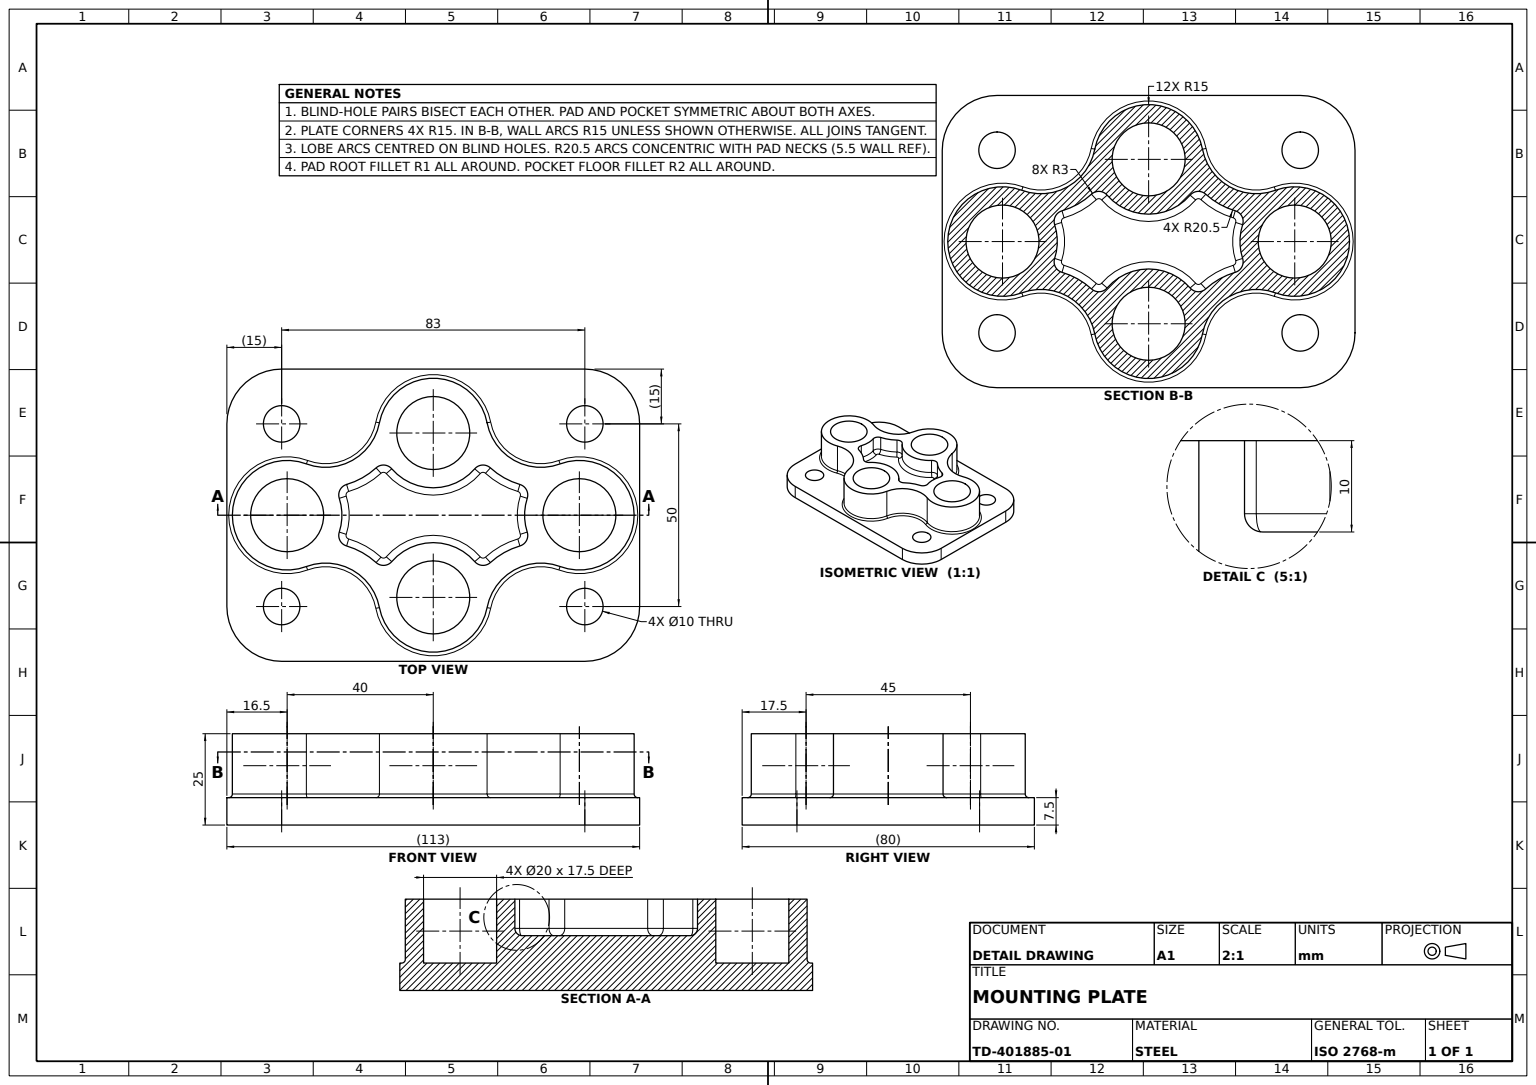
solid
v1 (14.982821,-34.38617,7.5)
v2 (-14.982821,-34.38617,7.5)
e1 v1 v2 CIRCLE(AX(P(0,-40,7.5),D(0,0,1),D(1,0,0)),16) rev
v3 (14.046394,-34.737034,8.5)
e2 v1 v3 CIRCLE(AX(P(14.982821,-34.38617,8.5),D(-0.350864382,0.936426284,0),D(-0.936426284,-0.350864382,0)),1)
v4 (-14.046394,-34.737034,8.5)
e3 v4 v3 CIRCLE(AX(P(0,-40,8.5),D(0,0,1),D(1,0,0)),15)
e4 v2 v4 CIRCLE(AX(P(-14.982821,-34.38617,8.5),D(-0.350864382,-0.936426284,0),D(0.936426284,-0.350864382,0)),1)
face TORUS(AX(P(0,-40,8.5),D(0,0,1),D(1,0,0)),16,1) rev [-e1 e2 -e3 -e4]
v5 (-40,41.5,7.5)
v6 (-40,-41.5,7.5)
e5 v5 v6 LINE
v7 (-40,41.5,0)
e6 v5 v7 LINE
v8 (-40,-41.5,0)
e7 v7 v8 LINE
e8 v8 v6 LINE
face PLANE(AX(P(-40,56.5,7.5),D(1,0,0),D(0,1,0))) rev [-e5 e6 e7 e8]
v9 (40,41.5,7.5)
v10 (25,56.5,7.5)
e9 v9 v10 CIRCLE(AX(P(25,41.5,7.5),D(0,0,1),D(1,0,0)),15)
v11 (40,41.5,0)
e10 v11 v9 LINE
v12 (25,56.5,0)
e11 v12 v11 CIRCLE(AX(P(25,41.5,0),D(0,0,1),D(1,0,0)),15) rev
e12 v10 v12 LINE
face CYL(AX(P(25,41.5,7.5),D(0,0,-1),D(-1,0,0)),15) [-e9 -e10 -e11 -e12]
v13 (-25.296394,-14.737034,8.5)
e13 v13 v4 CIRCLE(AX(P(-28.092789,-29.474069,8.5),D(0,0,1),D(1,0,0)),15) rev
v14 (-14.046394,-34.737034,25)
e14 v14 v4 LINE
v15 (-25.296394,-14.737034,25)
e15 v15 v14 CIRCLE(AX(P(-28.092789,-29.474069,25),D(0,0,-1),D(1,0,0)),15)
e16 v15 v13 LINE
face CYL(AX(P(-28.092789,-29.474069,25),D(0,0,-1),D(-1,0,0)),15) rev [e13 -e14 -e15 e16]
v16 (14.046394,-34.737034,25)
e17 v16 v3 LINE
e18 v14 v16 CIRCLE(AX(P(0,-40,25),D(0,0,1),D(1,0,0)),15)
face CYL(AX(P(0,-40,25),D(0,0,-1),D(-1,0,0)),15) [-e17 -e18 e14 e3]
v17 (-5.231122,23.824853,15)
v18 (-4.615696,25.727812,17)
e19 v17 v18 CIRCLE(AX(P(-5.231122,23.824853,17),D(0.95147921,-0.307713037,0),D(0.307713037,0.95147921,0)),2)
v19 (5.231122,23.824853,15)
e20 v19 v17 CIRCLE(AX(P(0,40,15),D(0,0,1),D(1,0,0)),17) rev
v20 (4.615696,25.727812,17)
e21 v19 v20 CIRCLE(AX(P(5.231122,23.824853,17),D(0.95147921,0.307713037,0),D(-0.307713037,0.95147921,0)),2)
e22 v18 v20 CIRCLE(AX(P(0,40,17),D(0,0,1),D(1,0,0)),15)
face TORUS(AX(P(0,40,17),D(0,0,1),D(1,0,0)),17,2) rev [-e19 -e20 e21 -e22]
v21 (-12.699871,11.355944,17)
v22 (-12.955115,15.650146,17)
e23 v21 v22 CIRCLE(AX(P(-10.739845,13.627133,17),D(0,0,1),D(1,0,0)),3) rev
v23 (-11.393187,12.87007,15)
e24 v23 v21 CIRCLE(AX(P(-11.393187,12.87007,17),D(-0.757062957,0.653341932,0),D(-0.653341932,-0.757062957,0)),2)
v24 (-11.478268,14.301471,15)
e25 v24 v23 CIRCLE(AX(P(-10.739845,13.627133,15),D(0,0,1),D(1,0,0)),1)
e26 v24 v22 CIRCLE(AX(P(-11.478268,14.301471,17),D(0.674337673,0.738423119,0),D(-0.738423119,0.674337673,0)),2)
face DEGENERATE_TOROIDAL_SURFACE(AX(P(-10.739845,13.627133,17),D(0,0,1),D(1,0,0)),1,2,.T.) rev [-e23 -e24 -e25 e26]
v25 (12.955115,-15.650146,17)
v26 (12.955115,-15.650146,25)
e27 v25 v26 LINE
v27 (12.699871,-11.355944,25)
e28 v27 v26 CIRCLE(AX(P(10.739845,-13.627133,25),D(0,0,1),D(1,0,0)),3) rev
v28 (12.699871,-11.355944,17)
e29 v28 v27 LINE
e30 v28 v25 CIRCLE(AX(P(10.739845,-13.627133,17),D(0,0,1),D(1,0,0)),3) rev
face CYL(AX(P(10.739845,-13.627133,43),D(0,0,-1),D(-1,0,0)),3) rev [e27 -e28 -e29 e30]
v29 (20,-41.5,7.5)
e31 v29 v29 CIRCLE(AX(P(25,-41.5,7.5),D(0,0,-1),D(-1,0,0)),5)
v30 (30,-41.5,0)
e32 v30 v30 CIRCLE(AX(P(25,-41.5,0),D(0,0,1),D(1,0,0)),5)
face CYL(AX(P(25,-41.5,7.5),D(0,0,-1),D(-1,0,0)),5) rev [-e31] [-e32]
v31 (25,-56.5,7.5)
v32 (40,-41.5,7.5)
e33 v31 v32 CIRCLE(AX(P(25,-41.5,7.5),D(0,0,1),D(1,0,0)),15)
v33 (25,-56.5,0)
e34 v33 v31 LINE
v34 (40,-41.5,0)
e35 v34 v33 CIRCLE(AX(P(25,-41.5,0),D(0,0,1),D(1,0,0)),15) rev
e36 v32 v34 LINE
face CYL(AX(P(25,-41.5,7.5),D(0,0,-1),D(-1,0,0)),15) [-e33 -e34 -e35 -e36]
v35 (-8.418063,-23.716016,17)
v36 (-12.955115,-15.650146,17)
e37 v35 v36 CIRCLE(AX(P(-28.092789,-29.474069,17),D(0,0,1),D(1,0,0)),20.5)
v37 (-6.498577,-23.154255,15)
e38 v35 v37 CIRCLE(AX(P(-6.498577,-23.154255,17),D(0.280880609,-0.959742717,0),D(0.959742717,0.280880609,0)),2)
v38 (-11.478268,-14.301471,15)
e39 v38 v37 CIRCLE(AX(P(-28.092789,-29.474069,15),D(0,0,1),D(1,0,0)),22.5) rev
e40 v36 v38 CIRCLE(AX(P(-11.478268,-14.301471,17),D(0.674337673,-0.738423119,0),D(0.738423119,0.674337673,0)),2)
face TORUS(AX(P(-28.092789,-29.474069,17),D(0,0,1),D(1,0,0)),22.5,2) rev [-e37 e38 -e39 -e40]
v39 (8.418063,-23.716016,17)
v40 (4.615696,-25.727812,17)
e41 v39 v40 CIRCLE(AX(P(5.538835,-22.873374,17),D(0,0,1),D(1,0,0)),3) rev
v41 (4.615696,-25.727812,25)
e42 v40 v41 LINE
v42 (8.418063,-23.716016,25)
e43 v42 v41 CIRCLE(AX(P(5.538835,-22.873374,25),D(0,0,1),D(1,0,0)),3) rev
e44 v39 v42 LINE
face CYL(AX(P(5.538835,-22.873374,43),D(0,0,-1),D(-1,0,0)),3) rev [e41 e42 -e43 -e44]
v43 (25.482821,-15.719503,7.5)
e45 v43 v1 CIRCLE(AX(P(28.092789,-29.474069,7.5),D(0,0,1),D(1,0,0)),14)
v44 (25.296394,-14.737034,8.5)
e46 v43 v44 CIRCLE(AX(P(25.482821,-15.719503,8.5),D(0.982468951,0.186426284,0),D(-0.186426284,0.982468951,0)),1)
e47 v3 v44 CIRCLE(AX(P(28.092789,-29.474069,8.5),D(0,0,1),D(1,0,0)),15) rev
face TORUS(AX(P(28.092789,-29.474069,8.5),D(0,0,1),D(1,0,0)),14,1) rev [-e2 -e45 e46 -e47]
v45 (-25.482821,15.719503,7.5)
v46 (-14.982821,34.38617,7.5)
e48 v45 v46 CIRCLE(AX(P(-28.092789,29.474069,7.5),D(0,0,1),D(1,0,0)),14)
v47 (-25.296394,14.737034,8.5)
e49 v47 v45 CIRCLE(AX(P(-25.482821,15.719503,8.5),D(0.982468951,0.186426284,0),D(-0.186426284,0.982468951,0)),1)
v48 (-14.046394,34.737034,8.5)
e50 v48 v47 CIRCLE(AX(P(-28.092789,29.474069,8.5),D(0,0,1),D(1,0,0)),15) rev
e51 v48 v46 CIRCLE(AX(P(-14.982821,34.38617,8.5),D(-0.350864382,0.936426284,0),D(-0.936426284,-0.350864382,0)),1)
face TORUS(AX(P(-28.092789,29.474069,8.5),D(0,0,1),D(1,0,0)),14,1) rev [-e48 -e49 -e50 e51]
v49 (30,41.5,0)
e52 v49 v49 CIRCLE(AX(P(25,41.5,0),D(0,0,1),D(1,0,0)),5)
v50 (20,41.5,7.5)
e53 v50 v50 CIRCLE(AX(P(25,41.5,7.5),D(0,0,-1),D(-1,0,0)),5)
face CYL(AX(P(25,41.5,7.5),D(0,0,-1),D(-1,0,0)),5) rev [-e52] [-e53]
v51 (-11.393187,-12.87007,15)
e54 v51 v38 CIRCLE(AX(P(-10.739845,-13.627133,15),D(0,0,1),D(1,0,0)),1)
v52 (-12.699871,-11.355944,17)
e55 v51 v52 CIRCLE(AX(P(-11.393187,-12.87007,17),D(0.757062957,0.653341932,0),D(-0.653341932,0.757062957,0)),2)
e56 v36 v52 CIRCLE(AX(P(-10.739845,-13.627133,17),D(0,0,1),D(1,0,0)),3) rev
face DEGENERATE_TOROIDAL_SURFACE(AX(P(-10.739845,-13.627133,17),D(0,0,1),D(1,0,0)),1,2,.T.) rev [e40 -e54 e55 -e56]
v53 (14.982821,34.38617,7.5)
v54 (25.482821,15.719503,7.5)
e57 v53 v54 CIRCLE(AX(P(28.092789,29.474069,7.5),D(0,0,1),D(1,0,0)),14)
v55 (14.046394,34.737034,8.5)
e58 v55 v53 CIRCLE(AX(P(14.982821,34.38617,8.5),D(-0.350864382,-0.936426284,0),D(0.936426284,-0.350864382,0)),1)
v56 (25.296394,14.737034,8.5)
e59 v56 v55 CIRCLE(AX(P(28.092789,29.474069,8.5),D(0,0,1),D(1,0,0)),15) rev
e60 v54 v56 CIRCLE(AX(P(25.482821,15.719503,8.5),D(-0.982468951,0.186426284,0),D(-0.186426284,-0.982468951,0)),1)
face TORUS(AX(P(28.092789,29.474069,8.5),D(0,0,1),D(1,0,0)),14,1) rev [-e57 -e58 -e59 -e60]
v57 (-8.418063,23.716016,17)
e61 v57 v18 CIRCLE(AX(P(-5.538835,22.873374,17),D(0,0,1),D(1,0,0)),3) rev
v58 (-6.498577,23.154255,15)
e62 v58 v57 CIRCLE(AX(P(-6.498577,23.154255,17),D(0.280880609,0.959742717,0),D(-0.959742717,0.280880609,0)),2)
e63 v17 v58 CIRCLE(AX(P(-5.538835,22.873374,15),D(0,0,1),D(1,0,0)),1)
face DEGENERATE_TOROIDAL_SURFACE(AX(P(-5.538835,22.873374,17),D(0,0,1),D(1,0,0)),1,2,.T.) rev [e19 -e61 -e62 -e63]
v59 (-25.296394,14.737034,25)
e64 v59 v15 CIRCLE(AX(P(-22.5,0,25),D(0,0,1),D(1,0,0)),15)
e65 v59 v47 LINE
e66 v47 v13 CIRCLE(AX(P(-22.5,0,8.5),D(0,0,1),D(1,0,0)),15)
face CYL(AX(P(-22.5,0,25),D(0,0,-1),D(-1,0,0)),15) [-e64 e65 e66 -e16]
v60 (-25,56.5,0)
e67 v7 v60 CIRCLE(AX(P(-25,41.5,0),D(0,0,1),D(1,0,0)),15) rev
v61 (-25,56.5,7.5)
e68 v61 v5 CIRCLE(AX(P(-25,41.5,7.5),D(0,0,1),D(1,0,0)),15)
e69 v60 v61 LINE
face CYL(AX(P(-25,41.5,7.5),D(0,0,-1),D(-1,0,0)),15) [-e67 -e6 -e68 -e69]
v62 (12.699871,11.355944,17)
e70 v62 v28 CIRCLE(AX(P(22.5,0,17),D(0,0,1),D(1,0,0)),15)
v63 (12.699871,11.355944,25)
e71 v63 v27 CIRCLE(AX(P(22.5,0,25),D(0,0,1),D(1,0,0)),15)
e72 v62 v63 LINE
face CYL(AX(P(22.5,0,43),D(0,0,-1),D(-1,0,0)),15) [e70 e29 -e71 -e72]
v64 (-25,-56.5,7.5)
v65 (-25,-56.5,0)
e73 v64 v65 LINE
e74 v65 v33 LINE
e75 v64 v31 LINE
face PLANE(AX(P(-40,-56.5,7.5),D(0,1,0),D(0,0,1))) rev [e73 e74 e34 -e75]
e76 v10 v61 LINE
e77 v12 v60 LINE
face PLANE(AX(P(40,56.5,7.5),D(0,-1,0),D(0,0,-1))) rev [-e76 e12 e77 e69]
v66 (-20,-41.5,0)
e78 v66 v66 CIRCLE(AX(P(-25,-41.5,0),D(0,0,1),D(1,0,0)),5)
v67 (-20,41.5,0)
e79 v67 v67 CIRCLE(AX(P(-25,41.5,0),D(0,0,1),D(1,0,0)),5)
e80 v34 v11 LINE
e81 v65 v8 CIRCLE(AX(P(-25,-41.5,0),D(0,0,1),D(1,0,0)),15) rev
face PLANE(AX(P(-25.296394,-14.737034,0),D(0,0,1),D(1,0,0))) rev [e78] [e52] [e32] [e79] [e11 -e80 e35 -e74 e81 -e7 e67 -e77]
v68 (-10,-40,7.5)
e82 v68 v68 CIRCLE(AX(P(0,-40,7.5),D(0,0,-1),D(-1,0,0)),10) rev
face PLANE(AX(P(0,-40,7.5),D(0,0,-1),D(-1,0,0))) rev [e82]
v69 (-4.615696,25.727812,25)
v70 (4.615696,25.727812,25)
e83 v69 v70 CIRCLE(AX(P(0,40,25),D(0,0,1),D(1,0,0)),15)
e84 v18 v69 LINE
e85 v20 v70 LINE
face CYL(AX(P(0,40,43),D(0,0,-1),D(-1,0,0)),15) [-e83 -e84 e22 e85]
v71 (12.955115,15.650146,17)
e86 v71 v62 CIRCLE(AX(P(10.739845,13.627133,17),D(0,0,1),D(1,0,0)),3) rev
v72 (12.955115,15.650146,25)
e87 v72 v63 CIRCLE(AX(P(10.739845,13.627133,25),D(0,0,1),D(1,0,0)),3) rev
e88 v71 v72 LINE
face CYL(AX(P(10.739845,13.627133,43),D(0,0,-1),D(-1,0,0)),3) rev [e86 e72 -e87 -e88]
v73 (25.296394,14.737034,25)
v74 (14.046394,34.737034,25)
e89 v73 v74 CIRCLE(AX(P(28.092789,29.474069,25),D(0,0,-1),D(1,0,0)),15)
e90 v73 v56 LINE
e91 v74 v55 LINE
face CYL(AX(P(28.092789,29.474069,25),D(0,0,-1),D(-1,0,0)),15) rev [-e89 e90 e59 -e91]
v75 (8.418063,23.716016,25)
e92 v75 v72 CIRCLE(AX(P(28.092789,29.474069,25),D(0,0,1),D(1,0,0)),20.5)
v76 (8.418063,23.716016,17)
e93 v76 v75 LINE
e94 v76 v71 CIRCLE(AX(P(28.092789,29.474069,17),D(0,0,1),D(1,0,0)),20.5)
face CYL(AX(P(28.092789,29.474069,43),D(0,0,-1),D(-1,0,0)),20.5) [-e92 -e93 e94 e88]
v77 (-25.482821,-15.719503,7.5)
e95 v13 v77 CIRCLE(AX(P(-25.482821,-15.719503,8.5),D(-0.982468951,0.186426284,0),D(-0.186426284,-0.982468951,0)),1)
e96 v2 v77 CIRCLE(AX(P(-28.092789,-29.474069,7.5),D(0,0,1),D(1,0,0)),14)
face TORUS(AX(P(-28.092789,-29.474069,8.5),D(0,0,1),D(1,0,0)),14,1) rev [e4 -e13 e95 -e96]
v78 (-4.615696,-25.727812,17)
v79 (-4.615696,-25.727812,25)
e97 v78 v79 LINE
e98 v41 v79 CIRCLE(AX(P(0,-40,25),D(0,0,1),D(1,0,0)),15)
e99 v40 v78 CIRCLE(AX(P(0,-40,17),D(0,0,1),D(1,0,0)),15)
face CYL(AX(P(0,-40,43),D(0,0,-1),D(-1,0,0)),15) [e97 -e98 -e42 e99]
e100 v77 v45 CIRCLE(AX(P(-22.5,0,7.5),D(0,0,1),D(1,0,0)),16) rev
face TORUS(AX(P(-22.5,0,8.5),D(0,0,1),D(1,0,0)),16,1) rev [-e66 e49 -e100 -e95]
v80 (-32.5,0,7.5)
e101 v80 v80 CIRCLE(AX(P(-22.5,0,7.5),D(0,0,-1),D(-1,0,0)),10) rev
face PLANE(AX(P(-22.5,0,7.5),D(0,0,-1),D(-1,0,0))) rev [e101]
v81 (-12.955115,-15.650146,25)
v82 (-12.699871,-11.355944,25)
e102 v81 v82 CIRCLE(AX(P(-10.739845,-13.627133,25),D(0,0,1),D(1,0,0)),3) rev
e103 v36 v81 LINE
e104 v52 v82 LINE
face CYL(AX(P(-10.739845,-13.627133,43),D(0,0,-1),D(-1,0,0)),3) rev [-e102 -e103 e56 e104]
v83 (6.498577,-23.154255,15)
e105 v39 v83 CIRCLE(AX(P(6.498577,-23.154255,17),D(0.280880609,0.959742717,0),D(-0.959742717,0.280880609,0)),2)
e106 v25 v39 CIRCLE(AX(P(28.092789,-29.474069,17),D(0,0,1),D(1,0,0)),20.5)
v84 (11.478268,-14.301471,15)
e107 v25 v84 CIRCLE(AX(P(11.478268,-14.301471,17),D(0.674337673,0.738423119,0),D(-0.738423119,0.674337673,0)),2)
e108 v83 v84 CIRCLE(AX(P(28.092789,-29.474069,15),D(0,0,1),D(1,0,0)),22.5) rev
face TORUS(AX(P(28.092789,-29.474069,17),D(0,0,1),D(1,0,0)),22.5,2) rev [-e105 -e106 e107 -e108]
v85 (12.5,0,7.5)
e109 v85 v85 CIRCLE(AX(P(22.5,0,7.5),D(0,0,-1),D(-1,0,0)),10) rev
face PLANE(AX(P(22.5,0,7.5),D(0,0,-1),D(-1,0,0))) rev [e109]
e110 v20 v76 CIRCLE(AX(P(5.538835,22.873374,17),D(0,0,1),D(1,0,0)),3) rev
e111 v70 v75 CIRCLE(AX(P(5.538835,22.873374,25),D(0,0,1),D(1,0,0)),3) rev
face CYL(AX(P(5.538835,22.873374,43),D(0,0,-1),D(-1,0,0)),3) rev [-e85 e110 e93 -e111]
v86 (-10,40,7.5)
e112 v86 v86 CIRCLE(AX(P(0,40,7.5),D(0,0,-1),D(-1,0,0)),10) rev
face PLANE(AX(P(0,40,7.5),D(0,0,-1),D(-1,0,0))) rev [e112]
v87 (6.498577,23.154255,15)
e113 v87 v76 CIRCLE(AX(P(6.498577,23.154255,17),D(0.280880609,-0.959742717,0),D(0.959742717,0.280880609,0)),2)
e114 v87 v19 CIRCLE(AX(P(5.538835,22.873374,15),D(0,0,1),D(1,0,0)),1)
face DEGENERATE_TOROIDAL_SURFACE(AX(P(5.538835,22.873374,17),D(0,0,1),D(1,0,0)),1,2,.T.) rev [e113 -e110 -e21 -e114]
v88 (-14.046394,34.737034,25)
e115 v88 v48 LINE
e116 v74 v88 CIRCLE(AX(P(0,40,25),D(0,0,1),D(1,0,0)),15)
e117 v55 v48 CIRCLE(AX(P(0,40,8.5),D(0,0,1),D(1,0,0)),15)
face CYL(AX(P(0,40,25),D(0,0,-1),D(-1,0,0)),15) [-e115 -e116 e91 e117]
v89 (-8.418063,23.716016,25)
e118 v57 v89 LINE
e119 v89 v69 CIRCLE(AX(P(-5.538835,22.873374,25),D(0,0,1),D(1,0,0)),3) rev
face CYL(AX(P(-5.538835,22.873374,43),D(0,0,-1),D(-1,0,0)),3) rev [-e118 e61 e84 -e119]
e120 v52 v21 CIRCLE(AX(P(-22.5,0,17),D(0,0,1),D(1,0,0)),15)
v90 (-12.699871,11.355944,25)
e121 v21 v90 LINE
e122 v82 v90 CIRCLE(AX(P(-22.5,0,25),D(0,0,1),D(1,0,0)),15)
face CYL(AX(P(-22.5,0,43),D(0,0,-1),D(-1,0,0)),15) [e120 e121 -e122 -e104]
v91 (-12.955115,15.650146,25)
e123 v90 v91 CIRCLE(AX(P(-10.739845,13.627133,25),D(0,0,1),D(1,0,0)),3) rev
e124 v22 v91 LINE
face CYL(AX(P(-10.739845,13.627133,43),D(0,0,-1),D(-1,0,0)),3) rev [-e123 -e121 e23 e124]
e125 v22 v57 CIRCLE(AX(P(-28.092789,29.474069,17),D(0,0,1),D(1,0,0)),20.5)
e126 v91 v89 CIRCLE(AX(P(-28.092789,29.474069,25),D(0,0,1),D(1,0,0)),20.5)
face CYL(AX(P(-28.092789,29.474069,43),D(0,0,-1),D(-1,0,0)),20.5) [e125 e118 -e126 -e124]
e127 v88 v59 CIRCLE(AX(P(-28.092789,29.474069,25),D(0,0,-1),D(1,0,0)),15)
face CYL(AX(P(-28.092789,29.474069,25),D(0,0,-1),D(-1,0,0)),15) rev [-e127 e115 e50 -e65]
v92 (-32.5,0,25)
e128 v92 v92 CIRCLE(AX(P(-22.5,0,25),D(0,0,-1),D(-1,0,0)),10)
v93 (12.5,0,25)
e129 v93 v93 CIRCLE(AX(P(22.5,0,25),D(0,0,-1),D(-1,0,0)),10)
v94 (-10,40,25)
e130 v94 v94 CIRCLE(AX(P(0,40,25),D(0,0,-1),D(-1,0,0)),10)
v95 (25.296394,-14.737034,25)
e131 v16 v95 CIRCLE(AX(P(28.092789,-29.474069,25),D(0,0,-1),D(1,0,0)),15)
e132 v95 v73 CIRCLE(AX(P(22.5,0,25),D(0,0,1),D(1,0,0)),15)
e133 v26 v42 CIRCLE(AX(P(28.092789,-29.474069,25),D(0,0,1),D(1,0,0)),20.5)
v96 (-8.418063,-23.716016,25)
e134 v79 v96 CIRCLE(AX(P(-5.538835,-22.873374,25),D(0,0,1),D(1,0,0)),3) rev
e135 v96 v81 CIRCLE(AX(P(-28.092789,-29.474069,25),D(0,0,1),D(1,0,0)),20.5)
v97 (-10,-40,25)
e136 v97 v97 CIRCLE(AX(P(0,-40,25),D(0,0,-1),D(-1,0,0)),10)
face PLANE(AX(P(-25.296394,-14.737034,25),D(0,0,1),D(1,0,0))) [e128] [e129] [e130] [e89 e116 e127 e64 e15 e18 e131 e132] [e126 e119 e83 e111 e92 e87 e71 e28 e133 e43 e98 e134 e135 e102 e122 e123] [e136]
v98 (11.393187,-12.87007,15)
e137 v28 v98 CIRCLE(AX(P(11.393187,-12.87007,17),D(-0.757062957,0.653341932,0),D(-0.653341932,-0.757062957,0)),2)
e138 v84 v98 CIRCLE(AX(P(10.739845,-13.627133,15),D(0,0,1),D(1,0,0)),1)
face DEGENERATE_TOROIDAL_SURFACE(AX(P(10.739845,-13.627133,17),D(0,0,1),D(1,0,0)),1,2,.T.) rev [-e107 -e30 e137 -e138]
e139 v46 v53 CIRCLE(AX(P(0,40,7.5),D(0,0,1),D(1,0,0)),16) rev
face TORUS(AX(P(0,40,8.5),D(0,0,1),D(1,0,0)),16,1) rev [e58 -e139 -e51 -e117]
face CYL(AX(P(22.5,0,25),D(0,0,-1),D(-1,0,0)),10) rev [-e129] [-e109]
v99 (11.393187,12.87007,15)
e140 v62 v99 CIRCLE(AX(P(11.393187,12.87007,17),D(0.757062957,0.653341932,0),D(-0.653341932,0.757062957,0)),2)
v100 (11.478268,14.301471,15)
e141 v100 v71 CIRCLE(AX(P(11.478268,14.301471,17),D(0.674337673,-0.738423119,0),D(0.738423119,0.674337673,0)),2)
e142 v99 v100 CIRCLE(AX(P(10.739845,13.627133,15),D(0,0,1),D(1,0,0)),1)
face DEGENERATE_TOROIDAL_SURFACE(AX(P(10.739845,13.627133,17),D(0,0,1),D(1,0,0)),1,2,.T.) rev [-e140 -e86 -e141 -e142]
v101 (-30,-41.5,7.5)
e143 v101 v101 CIRCLE(AX(P(-25,-41.5,7.5),D(0,0,-1),D(-1,0,0)),5)
face CYL(AX(P(-25,-41.5,7.5),D(0,0,-1),D(-1,0,0)),5) rev [-e143] [-e78]
e144 v58 v24 CIRCLE(AX(P(-28.092789,29.474069,15),D(0,0,1),D(1,0,0)),22.5) rev
face TORUS(AX(P(-28.092789,29.474069,17),D(0,0,1),D(1,0,0)),22.5,2) rev [e62 -e125 -e26 -e144]
e145 v98 v99 CIRCLE(AX(P(22.5,0,15),D(0,0,1),D(1,0,0)),17) rev
face TORUS(AX(P(22.5,0,17),D(0,0,1),D(1,0,0)),17,2) rev [e140 -e145 -e137 -e70]
face CYL(AX(P(-22.5,0,25),D(0,0,-1),D(-1,0,0)),10) rev [-e128] [-e101]
e146 v6 v64 CIRCLE(AX(P(-25,-41.5,7.5),D(0,0,1),D(1,0,0)),15)
e147 v32 v9 LINE
e148 v54 v43 CIRCLE(AX(P(22.5,0,7.5),D(0,0,1),D(1,0,0)),16) rev
v102 (-30,41.5,7.5)
e149 v102 v102 CIRCLE(AX(P(-25,41.5,7.5),D(0,0,-1),D(-1,0,0)),5)
face PLANE(AX(P(0,0,7.5),D(0,0,1),D(1,0,0))) [e31] [e146 e75 e33 e147 e9 e76 e68 e5] [e53] [e96 e100 e48 e139 e57 e148 e45 e1] [e143] [e149]
e150 v100 v87 CIRCLE(AX(P(28.092789,29.474069,15),D(0,0,1),D(1,0,0)),22.5) rev
face TORUS(AX(P(28.092789,29.474069,17),D(0,0,1),D(1,0,0)),22.5,2) rev [-e113 -e150 e141 -e94]
face CYL(AX(P(-25,-41.5,7.5),D(0,0,-1),D(-1,0,0)),15) [-e81 -e73 -e146 -e8]
e151 v23 v51 CIRCLE(AX(P(-22.5,0,15),D(0,0,1),D(1,0,0)),17) rev
v103 (-5.231122,-23.824853,15)
e152 v37 v103 CIRCLE(AX(P(-5.538835,-22.873374,15),D(0,0,1),D(1,0,0)),1)
v104 (5.231122,-23.824853,15)
e153 v103 v104 CIRCLE(AX(P(0,-40,15),D(0,0,1),D(1,0,0)),17) rev
e154 v104 v83 CIRCLE(AX(P(5.538835,-22.873374,15),D(0,0,1),D(1,0,0)),1)
face PLANE(AX(P(-19.416317,-21.550601,15),D(0,0,1),D(1,0,0))) [e151 e54 e39 e152 e153 e154 e108 e138 e145 e142 e150 e114 e20 e63 e144 e25]
e155 v78 v35 CIRCLE(AX(P(-5.538835,-22.873374,17),D(0,0,1),D(1,0,0)),3) rev
e156 v35 v96 LINE
face CYL(AX(P(-5.538835,-22.873374,43),D(0,0,-1),D(-1,0,0)),3) rev [-e97 e155 e156 -e134]
e157 v44 v56 CIRCLE(AX(P(22.5,0,8.5),D(0,0,1),D(1,0,0)),15)
face TORUS(AX(P(22.5,0,8.5),D(0,0,1),D(1,0,0)),16,1) rev [-e46 -e148 e60 -e157]
face CYL(AX(P(-25,41.5,7.5),D(0,0,-1),D(-1,0,0)),5) rev [-e149] [-e79]
face TORUS(AX(P(-22.5,0,17),D(0,0,1),D(1,0,0)),17,2) rev [e24 -e120 -e55 -e151]
face PLANE(AX(P(40,-56.5,7.5),D(-1,0,0),D(0,0,1))) rev [e80 e10 -e147 e36]
face CYL(AX(P(-28.092789,-29.474069,43),D(0,0,-1),D(-1,0,0)),20.5) [-e135 -e156 e37 e103]
e158 v95 v44 LINE
face CYL(AX(P(28.092789,-29.474069,25),D(0,0,-1),D(-1,0,0)),15) rev [-e131 e17 e47 -e158]
face CYL(AX(P(28.092789,-29.474069,43),D(0,0,-1),D(-1,0,0)),20.5) [-e133 -e27 e106 e44]
face CYL(AX(P(0,-40,25),D(0,0,-1),D(-1,0,0)),10) rev [-e82] [-e136]
e159 v78 v103 CIRCLE(AX(P(-5.231122,-23.824853,17),D(0.95147921,0.307713037,0),D(-0.307713037,0.95147921,0)),2)
face DEGENERATE_TOROIDAL_SURFACE(AX(P(-5.538835,-22.873374,17),D(0,0,1),D(1,0,0)),1,2,.T.) rev [-e152 -e38 -e155 e159]
face CYL(AX(P(0,40,25),D(0,0,-1),D(-1,0,0)),10) rev [-e130] [-e112]
e160 v40 v104 CIRCLE(AX(P(5.231122,-23.824853,17),D(0.95147921,-0.307713037,0),D(0.307713037,0.95147921,0)),2)
face TORUS(AX(P(0,-40,17),D(0,0,1),D(1,0,0)),17,2) rev [-e153 -e159 -e99 e160]
face DEGENERATE_TOROIDAL_SURFACE(AX(P(5.538835,-22.873374,17),D(0,0,1),D(1,0,0)),1,2,.T.) rev [-e160 -e41 e105 -e154]
face CYL(AX(P(22.5,0,25),D(0,0,-1),D(-1,0,0)),15) [-e90 -e132 e158 e157]
